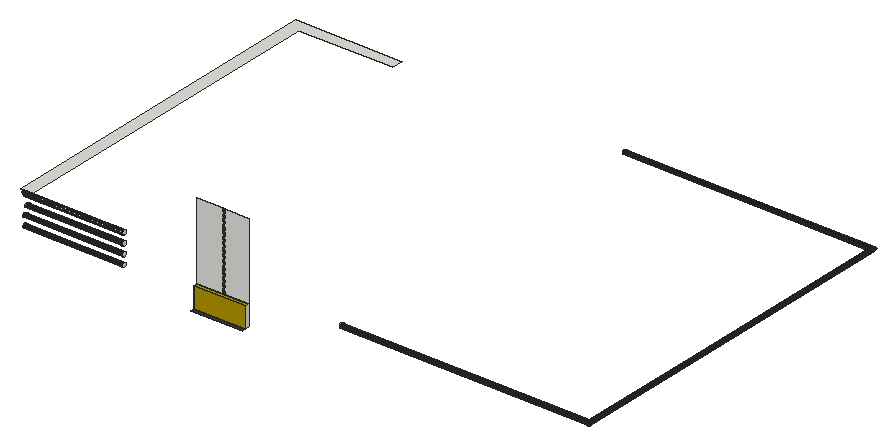
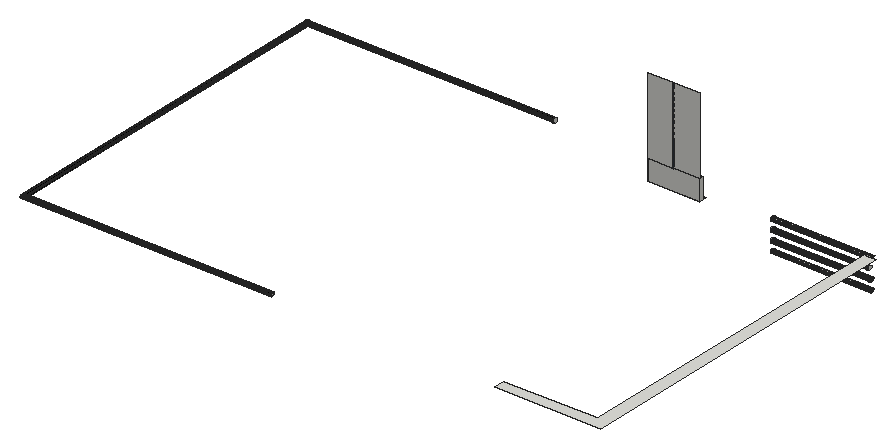
# SketchUp Ruby script. Lengths in inches.
U = 1.inch
M = Sketchup.active_model
def pt(a) = Geom::Point3d.new(a.map { |v| v * U })
def face(e, loops, mat)
  f = e.add_face(loops[0].map { |a| pt(a) })
  loops[1..].each { |l| e.add_face(l.map { |a| pt(a) }).erase! }
  f.material = f.back_material = mat if mat
  f
end
# faces: each face lists its corners as indices into pts; further lists are holes
def faces(e, pts, list, mat = nil) = list.each { |f| face(e, (f[0].is_a?(Array) ? f : [f]).map { |l| l.map { |i| pts[i] } }, mat) }
# xy, xz, yz: faces in a plane at the given z, y or x. An outline is a flat list of corners, or four numbers for a rectangle; further outlines are holes
def ring(l) = l.size == 4 ? [[l[0], l[1]], [l[2], l[1]], [l[2], l[3]], [l[0], l[3]]] : l.each_slice(2).to_a
def flat(e, list, mat, &to3) = list.each { |f| face(e, (f[0].is_a?(Array) ? f : [f]).map { |l| ring(l).map { |u, v| to3.(u, v) } }, mat) }
def xy(e, z, list, mat = nil) = flat(e, list, mat) { |x, y| [x, y, z] }
def xz(e, y, list, mat = nil) = flat(e, list, mat) { |x, z| [x, y, z] }
def yz(e, x, list, mat = nil) = flat(e, list, mat) { |y, z| [x, y, z] }
def lines(e, pts, list) = list.each { |a, b| e.add_line(pt(pts[a]), pt(pts[b])) }
# prism: a flat outline (further loops are holes) pulled along v
def prism(e, loops, v, mat = nil)
  f = face(e, loops, mat); d = Geom::Vector3d.new(v.map { |x| x * U })
  f.pushpull(f.normal.samedirection?(d) ? d.length : -d.length)
end
def box(e, o, s, mat = nil) = prism(e, [[o, [o[0] + s[0], o[1], o[2]], [o[0] + s[0], o[1] + s[1], o[2]], [o[0], o[1] + s[1], o[2]]]], [0, 0, s[2]], mat)
def at(x, y, z, deg = 0) = Geom::Transformation.translation(pt([x, y, z])) * Geom::Transformation.rotation(ORIGIN, Z_AXIS, deg.degrees)
def axes(o, x, y, z) = Geom::Transformation.new([*x, 0, *y, 0, *z, 0, *pt(o).to_a, 1])
def part(name) = M.definitions.add(name)
# library, detail: a bought-in or finely detailed component or shape, given as its bounding box
def library(name, o, s) = part(name).tap { |d| box(d.entities, o, s) }
def detail(e, o, s) = box(e.add_group.entities, o, s)
def put(e, d, t, mat = nil) = e.add_instance(d, t).tap { |i| i.material = mat if mat }
def group(e, t, mat = nil) = e.add_group.tap { |g| g.transformation = t; g.material = mat if mat }.entities
root = M.entities
M.materials.add("[0046_Gold]").color = [178, 150, 0]
M.materials.add("[0111_SlateGray]").color = [51, 58, 66]
M.materials.add("[0137_Black]").color = [0, 0, 0]
prism(root,[[[162,147.78,690.375],[162,148.5,690.68],[162,149.12,691.15],[162,149.6,691.77],[162,149.9,692.5],[162,150,693.27],[162,149.9,694.05],[162,149.6,694.77],[162,149.12,695.4],[162,148.5,695.87],[162,147.78,696.17],[162,147,696.27],[162,146.22,696.17],[162,145.5,695.87],[162,144.88,695.4],[162,144.4,694.77],[162,144.1,694.05],[162,144,693.27],[162,144.1,692.5],[162,144.4,691.77],[162,144.88,691.15],[162,145.5,690.68],[162,146.22,690.375],[162,147,690.27]]],[-150.02,0,0])
xy(root,669.07,[[299.18,108,378.44,114]])
xy(root,669.07,[[299.18,102,378.44,108]],"[0111_SlateGray]")
xy(root,681.45,[[9,146.59,162,147.375]])
xy(root,700.42,[[299.18,108,378.44,114]],"[0046_Gold]")
xy(root,708.875,[[510,126.5,889,128.5],[889,126.5,891,669],[510,669,891,671]])
xy(root,709.65,[[0,149.68,18,149.68,18,660,162,660,162,678,0,678]])
xz(root,108,[[299.18,669.07,378.44,700.42]],"[0046_Gold]")
xz(root,114,[[299.18,669.07,378.44,700.42],[299.18,700.42,338.27,817.66],[341.81,700.42,378.44,817.66]])
xz(root,114,[[338.27,700.42,341.81,817.66]],"[0111_SlateGray]")
xz(root,126.5,[[510,708.875,891,711.875]])
xz(root,669,[[510,708.875,891,711.875]])
yz(root,9,[[147,660.68,146.89,660.7,147,660.7],[147,660.68,147,660.7,147.28,660.72],[146.5,660.75,146.22,660.78,146.12,660.83],[147.66,660.77,148.03,660.89,147.78,660.78],[145.76,660.98,145.5,661.08,145.41,661.15],
  [148.39,661.04,148.72,661.25,148.5,661.08],[145.1,661.39,144.88,661.5625,144.81,661.65],[149.03,661.49,149.29,661.78,149.12,661.5625],[144.57,661.96,144.4,662.18,144.36,662.29],[149.53,662.09,149.7,662.4375,149.6,662.18],
  [144.21,662.65,144.1,662.91,144.09,663.02],[149.85,662.8,149.93,663.18,149.9,662.91],[144.04,663.41,144,663.68,144.02,663.8],[149.98,663.57,149.96,663.96,150,663.68],[144.07,664.18,144.1,664.46,144.15,664.57],
  [149.91,664.34,149.79,664.72,149.9,664.46],[144.3,664.93,144.4,665.18,144.47,665.27],[149.64,665.08,149.43,665.4,149.6,665.18],[144.71,665.58,144.88,665.8,144.97,665.875],[149.19,665.71,148.9,665.97,149.12,665.8],
  [145.28,666.11,145.5,666.28,145.61,666.32],[148.59,666.21,148.24,666.39,148.5,666.28],[145.97,666.47,146.22,666.58,146.34,666.6],[147.88,666.54,147.5,666.62,147.78,666.58],[146.72,666.65,147,666.68,147,666.66],
  [147,666.66,147,666.68,147.11,666.67],[147,675.48,146.8125,675.5,147,675.5],[147,675.48,147,675.5,147.2,675.51],[146.43,675.55,146.22,675.58,146.05,675.65],[147.59,675.56,147.97,675.66,147.78,675.58],
  [145.69,675.8,145.5,675.88,145.35,675.99],[148.33,675.81,148.66,676.01,148.5,675.88],[145.04,676.23,144.88,676.36,144.76,676.51],[148.97,676.24,149.25,676.52,149.12,676.36],[144.53,676.82,144.4,676.98,144.33,677.15],
  [149.48,676.83,149.68,677.17,149.6,676.98],[144.18,677.51,144.1,677.7,144.08,677.89],[149.83,677.53,149.92,677.91,149.9,677.7],[144.03,678.27,144,678.48,144.02,678.66],[149.98,678.29,149.97,678.68,150,678.48],
  [144.08,679.05,144.1,679.25,144.17,679.43],[149.92,679.07,149.82,679.44,149.9,679.25],[144.32,679.79,144.4,679.98,144.52,680.13],[149.67,679.8,149.47,680.14,149.6,679.98],[144.75,680.4375,144.88,680.6,145.03,680.71],
  [149.24,680.45,148.96,680.72,149.12,680.6],[145.34,680.95,145.5,681.08,145.67,681.15],[148.65,680.96,148.31,681.16,148.5,681.08],[146.03,681.3,146.22,681.375,146.41,681.4],[147.95,681.3,147.57,681.4,147.78,681.375],
  [146.8,681.45,147,681.48,147,681.45],[147,681.45,147,681.48,147.1875,681.45]])
yz(root,162,[[146.77,660.69,146,660.85,145.31,661.21,144.72,661.73,144.29,662.39,144.05,663.13,144.01,663.91,144.17,664.68,144.52,665.375,145.05,665.96,145.7,666.39,146.45,666.63,147,666.66,147.23,666.67,148,666.51,148.69,666.16,149.28,665.64,149.71,664.98,149.95,664.24,149.99,663.45,149.83,662.6875,149.48,661.99,148.95,661.41,148.3,660.98,147.55,660.73,147,660.7],[146.625,675.5,145.87,675.7,145.1875,676.09,144.63,676.64,144.24,677.3125,144.03,678.07,144.02,678.85,144.22,679.61,144.61,680.29,145.16,680.85,145.84,681.24,146.59,681.45,147.375,681.45,148.13,681.26,148.8125,680.87,149.37,680.32,149.76,679.64,149.97,678.89,149.98,678.1,149.78,677.35,149.39,676.67,148.84,676.11,148.16,675.71,147.41,675.51,147,675.5],[146.82,705.01,147,705.02,147.6,705.0625,148.34,705.32,148.99,705.76,149.5,706.35,149.85,707.05,149.99,707.82,149.9375,708.6,149.68,709.34,149.24,709.99,148.65,710.5,147.95,710.85,147.18,710.99,146.4,710.9375,145.66,710.68,145.01,710.24,144.5,709.65,144.15,708.95,144.01,708.18,144.0625,707.4,144.32,706.66,144.76,706.01,145.35,705.5,146.05,705.15]])
yz(root,299.18,[[108,669.07,114,700.42]])
yz(root,378.44,[[108,669.07,114,700.42]])
yz(root,510,[[126.5,708.875,125.72,708.98,125,709.28,124.38,709.75,123.9,710.375,123.6,711.1,123.5,711.875,123.6,712.65,123.9,713.375,124.38,714,125,714.47,125.72,714.77,126.5,714.875,127.28,714.77,128,714.47,128.62,714,129.1,713.375,129.4,712.65,129.5,711.875,129.4,711.1,129.1,710.375,128.62,709.75,128,709.28,127.28,708.98]])
yz(root,891,[[126.5,708.875,669,711.875]])
p = [[162,146,660.85],[162,146.77,660.69],[9,146.77,660.69],[9,146.5,660.75],[9,146.12,660.83],[9,146,660.85],
  [162,147,660.7],[162,147.55,660.73],[9,147.55,660.73],[9,147.28,660.72],[9,147,660.7],[9,146.89,660.7],
  [162,148.3,660.98],[9,148.3,660.98],[9,148.03,660.89],[9,147.66,660.77],[162,145.31,661.21],[9,145.76,660.98],
  [9,145.41,661.15],[9,145.31,661.21],[162,148.95,661.41],[9,148.95,661.41],[9,148.72,661.25],[9,148.39,661.04],
  [162,144.72,661.73],[9,145.1,661.39],[9,144.81,661.65],[9,144.72,661.73],[162,149.48,661.99],[9,149.48,661.99],
  [9,149.29,661.78],[9,149.03,661.49],[162,144.29,662.39],[9,144.57,661.96],[9,144.36,662.29],[9,144.29,662.39],
  [162,149.83,662.6875],[9,149.83,662.6875],[9,149.7,662.4375],[9,149.53,662.09],[162,144.05,663.13],[9,144.21,662.65],
  [9,144.09,663.02],[9,144.05,663.13],[162,149.99,663.45],[9,149.99,663.45],[9,149.93,663.18],[9,149.85,662.8],
  [162,144.01,663.91],[9,144.04,663.41],[9,144.02,663.8],[9,144.01,663.91],[162,149.95,664.24],[9,149.95,664.24],
  [9,149.96,663.96],[9,149.98,663.57],[162,144.17,664.68],[9,144.07,664.18],[9,144.15,664.57],[9,144.17,664.68],
  [162,149.71,664.98],[9,149.71,664.98],[9,149.79,664.72],[9,149.91,664.34],[162,144.52,665.375],[9,144.3,664.93],
  [9,144.47,665.27],[9,144.52,665.375],[162,149.28,665.64],[9,149.28,665.64],[9,149.43,665.4],[9,149.64,665.08],
  [162,145.05,665.96],[9,144.71,665.58],[9,144.97,665.875],[9,145.05,665.96],[162,148.69,666.16],[9,148.69,666.16],
  [9,148.9,665.97],[9,149.19,665.71],[162,145.7,666.39],[9,145.28,666.11],[9,145.61,666.32],[9,145.7,666.39],
  [162,148,666.51],[9,148,666.51],[9,148.24,666.39],[9,148.59,666.21],[162,146.45,666.63],[9,145.97,666.47],
  [9,146.34,666.6],[9,146.45,666.63],[162,147.23,666.67],[9,147.23,666.67],[9,147.5,666.62],[9,147.88,666.54],
  [162,147,666.66],[9,146.72,666.65],[9,147,666.66],[9,147.11,666.67],[162,145.87,675.7],[162,146.625,675.5],
  [9,146.625,675.5],[9,146.43,675.55],[9,146.05,675.65],[9,145.87,675.7],[162,147,675.5],[162,147.41,675.51],
  [9,147.41,675.51],[9,147.2,675.51],[9,147,675.5],[9,146.8125,675.5],[162,148.16,675.71],[9,148.16,675.71],
  [9,147.97,675.66],[9,147.59,675.56],[162,145.1875,676.09],[9,145.69,675.8],[9,145.35,675.99],[9,145.1875,676.09],
  [162,148.84,676.11],[9,148.84,676.11],[9,148.66,676.01],[9,148.33,675.81],[162,144.63,676.64],[9,145.04,676.23],
  [9,144.76,676.51],[9,144.63,676.64],[162,149.39,676.67],[9,149.39,676.67],[9,149.25,676.52],[9,148.97,676.24],
  [162,144.24,677.3125],[9,144.53,676.82],[9,144.33,677.15],[9,144.24,677.3125],[162,149.78,677.35],[9,149.78,677.35],
  [9,149.68,677.17],[9,149.48,676.83],[162,144.03,678.07],[9,144.18,677.51],[9,144.08,677.89],[9,144.03,678.07],
  [162,149.98,678.1],[9,149.98,678.1],[9,149.92,677.91],[9,149.83,677.53],[162,144.02,678.85],[9,144.03,678.27],
  [9,144.02,678.66],[9,144.02,678.85],[162,149.97,678.89],[9,149.97,678.89],[9,149.97,678.68],[9,149.98,678.29],
  [162,144.22,679.61],[9,144.08,679.05],[9,144.17,679.43],[9,144.22,679.61],[162,149.76,679.64],[9,149.76,679.64],
  [9,149.82,679.44],[9,149.92,679.07],[162,144.61,680.29],[9,144.32,679.79],[9,144.52,680.13],[9,144.61,680.29],
  [162,149.37,680.32],[9,149.37,680.32],[9,149.47,680.14],[9,149.67,679.8],[162,145.16,680.85],[9,144.75,680.4375],
  [9,145.03,680.71],[9,145.16,680.85],[162,148.8125,680.87],[9,148.8125,680.87],[9,148.96,680.72],[9,149.24,680.45],
  [162,145.84,681.24],[9,145.34,680.95],[9,145.67,681.15],[9,145.84,681.24],[162,148.13,681.26],[9,148.13,681.26],
  [9,148.31,681.16],[9,148.65,680.96],[162,146.59,681.45],[9,146.03,681.3],[9,146.41,681.4],[9,146.59,681.45],
  [162,147.375,681.45],[9,147.375,681.45],[9,147.57,681.4],[9,147.95,681.3],[162,146.82,705.01],[162,146.05,705.15],
  [11.85,146.05,705.15],[11.99,146.82,705.01],[162,147.6,705.0625],[162,147,705.02],[11.98,147,705.02],[11.9375,147.6,705.0625],
  [162,148.34,705.32],[11.68,148.34,705.32],[162,145.35,705.5],[11.5,145.35,705.5],[162,148.99,705.76],[11.24,148.99,705.76],
  [162,144.76,706.01],[10.99,144.76,706.01],[162,149.5,706.35],[10.65,149.5,706.35],[162,144.32,706.66],[10.34,144.32,706.66],
  [162,149.85,707.05],[9.95,149.85,707.05],[162,144.0625,707.4],[9.6,144.0625,707.4],[162,149.99,707.82],[9.18,149.99,707.82],
  [162,144.01,708.18],[8.82,144.01,708.18],[162,149.9375,708.6],[8.4,149.9375,708.6],[162,144.15,708.95],[8.05,144.15,708.95],
  [162,149.68,709.34],[7.66,149.68,709.34],[18,149.68,709.34],[510,125.72,708.98],[510,126.5,708.875],[889,126.5,708.875],
  [891,126.5,708.875],[891.78,125.72,708.98],[891,669,708.875],[891.78,669.78,708.98],[510,127.28,708.98],[890.22,127.28,708.98],
  [890.22,668.22,708.98],[162,144.5,709.65],[7.35,144.5,709.65],[510,668.22,708.98],[510,669,708.875],[889,669,708.875],
  [510,669.78,708.98],[510,125,709.28],[892.5,125,709.28],[892.5,670.5,709.28],[510,128,709.28],[889.5,128,709.28],
  [889.5,667.5,709.28],[510,667.5,709.28],[510,670.5,709.28],[510,124.38,709.75],[893.12,124.38,709.75],[893.12,671.12,709.75],
  [510,128.62,709.75],[888.88,128.62,709.75],[888.88,666.88,709.75],[162,149.24,709.99],[7.01,149.24,709.99],[510,666.88,709.75],
  [510,671.12,709.75],[162,145.01,710.24],[6.76,145.01,710.24],[510,123.9,710.375],[893.6,123.9,710.375],[893.6,671.6,710.375],
  [510,129.1,710.375],[888.4,129.1,710.375],[888.4,666.4,710.375],[510,666.4,710.375],[510,671.6,710.375],[162,148.65,710.5],
  [6.5,148.65,710.5],[162,145.66,710.68],[6.32,145.66,710.68],[510,123.6,711.1],[893.9,123.6,711.1],[893.9,671.9,711.1],
  [510,129.4,711.1],[888.1,129.4,711.1],[888.1,666.1,711.1],[510,666.1,711.1],[510,671.9,711.1],[162,147.95,710.85],
  [6.15,147.95,710.85],[162,146.4,710.9375],[6.0625,146.4,710.9375],[162,147.18,710.99],[6.01,147.18,710.99],[510,123.5,711.875],
  [894,123.5,711.875],[894,672,711.875],[510,129.5,711.875],[888,129.5,711.875],[888,666,711.875],[510,666,711.875],
  [510,672,711.875],[510,123.6,712.65],[893.9,123.6,712.65],[893.9,671.9,712.65],[510,129.4,712.65],[888.1,129.4,712.65],
  [888.1,666.1,712.65],[510,666.1,712.65],[510,671.9,712.65],[510,123.9,713.375],[893.6,123.9,713.375],[893.6,671.6,713.375],
  [510,129.1,713.375],[888.4,129.1,713.375],[888.4,666.4,713.375],[510,666.4,713.375],[510,671.6,713.375],[510,124.38,714],
  [893.12,124.38,714],[893.12,671.12,714],[510,128.62,714],[888.88,128.62,714],[888.88,666.88,714],[510,666.88,714],
  [510,671.12,714],[510,125,714.47],[892.5,125,714.47],[892.5,670.5,714.47],[510,128,714.47],[889.5,128,714.47],
  [889.5,667.5,714.47],[510,667.5,714.47],[510,670.5,714.47],[510,125.72,714.77],[891.78,125.72,714.77],[891.78,669.78,714.77],
  [510,127.28,714.77],[890.22,127.28,714.77],[890.22,668.22,714.77],[510,668.22,714.77],[510,669.78,714.77],[510,126.5,714.875],
  [891,126.5,714.875],[891,669,714.875],[510,669,714.875],[9,147,708],[162,147,708],[9,147,663.68],
  [162,147,663.68],[9,147,681.48],[9,147,678.48],[162,147,678.48],[11.98,147,693.27],[162,147,693.27],
  [9,147,666.68],[9,147,675.48]]
faces(root,p,[[0,1,2,3,4,5],[6,7,8,9,10,11,2,1],[7,12,13,14,15,8],[16,0,5,17,18,19],[12,20,21,22,23,13],[24,16,19,25,26,27],[20,28,29,30,31,21],[32,24,27,33,34,35],
  [28,36,37,38,39,29],[40,32,35,41,42,43],[36,44,45,46,47,37],[48,40,43,49,50,51],[44,52,53,54,55,45],[56,48,51,57,58,59],[52,60,61,62,63,53],[64,56,59,65,66,67],
  [60,68,69,70,71,61],[72,64,67,73,74,75],[68,76,77,78,79,69],[80,72,75,81,82,83],[76,84,85,86,87,77],[88,80,83,89,90,91],[84,92,93,94,95,85],[96,88,91,97,98,99,93,92],
  [100,101,102,103,104,105],[106,107,108,109,110,111,102,101],[107,112,113,114,115,108],[116,100,105,117,118,119],[112,120,121,122,123,113],[124,116,119,125,126,127],[120,128,129,130,131,121],[132,124,127,133,134,135],
  [128,136,137,138,139,129],[140,132,135,141,142,143],[136,144,145,146,147,137],[148,140,143,149,150,151],[144,152,153,154,155,145],[156,148,151,157,158,159],[152,160,161,162,163,153],[164,156,159,165,166,167],
  [160,168,169,170,171,161],[172,164,167,173,174,175],[168,176,177,178,179,169],[180,172,175,181,182,183],[176,184,185,186,187,177],[188,180,183,189,190,191],[184,192,193,194,195,185],[196,197,198,199],
  [200,201,196,199,202,203],[204,200,203,205],[197,206,207,198],[208,204,205,209],[206,210,211,207],[212,208,209,213],[210,214,215,211],[216,212,213,217],
  [214,218,219,215],[220,216,217,221],[218,222,223,219],[224,220,221,225],[222,226,227,223],[228,224,225,229,230],[226,241,242,227],[261,228,230,229,262],
  [241,265,266,242],[275,261,262,276],[265,277,278,266],[287,275,276,288],[277,289,290,278],[291,287,288,292],[289,291,292,290]])
faces(root,p,[[231,232,233,234,235],[235,234,236,237],[232,238,239,234,233],[234,239,240,236],[236,240,243,244,245],[237,236,245,244,246],[247,231,235,248],[248,235,237,249],
  [238,250,251,239],[239,251,252,240],[240,252,253,243],[249,237,246,254],[255,247,248,256],[256,248,249,257],[250,258,259,251],[251,259,260,252],
  [252,260,263,253],[257,249,254,264],[267,255,256,268],[268,256,257,269],[258,270,271,259],[259,271,272,260],[260,272,273,263],[269,257,264,274],
  [279,267,268,280],[280,268,269,281],[270,282,283,271],[271,283,284,272],[272,284,285,273],[281,269,274,286],[293,279,280,294],[294,280,281,295],
  [282,296,297,283],[283,297,298,284],[284,298,299,285],[295,281,286,300],[301,293,294,302],[302,294,295,303],[296,304,305,297],[297,305,306,298],
  [298,306,307,299],[303,295,300,308],[309,301,302,310],[310,302,303,311],[304,312,313,305],[305,313,314,306],[306,314,315,307],[311,303,308,316],
  [317,309,310,318],[318,310,311,319],[312,320,321,313],[313,321,322,314],[314,322,323,315],[319,311,316,324],[325,317,318,326],[326,318,319,327],
  [320,328,329,321],[321,329,330,322],[322,330,331,323],[327,319,324,332],[333,325,326,334],[334,326,327,335],[328,336,337,329],[329,337,338,330],
  [330,338,339,331],[335,327,332,340],[341,333,334,342],[342,334,335,343],[336,341,342,337],[337,342,343,338],[338,343,344,339],[343,335,340,344]],"[0137_Black]")
lines(root,p,[[345,346],[347,348],[349,345],[350,351],[352,353],[354,355]])
